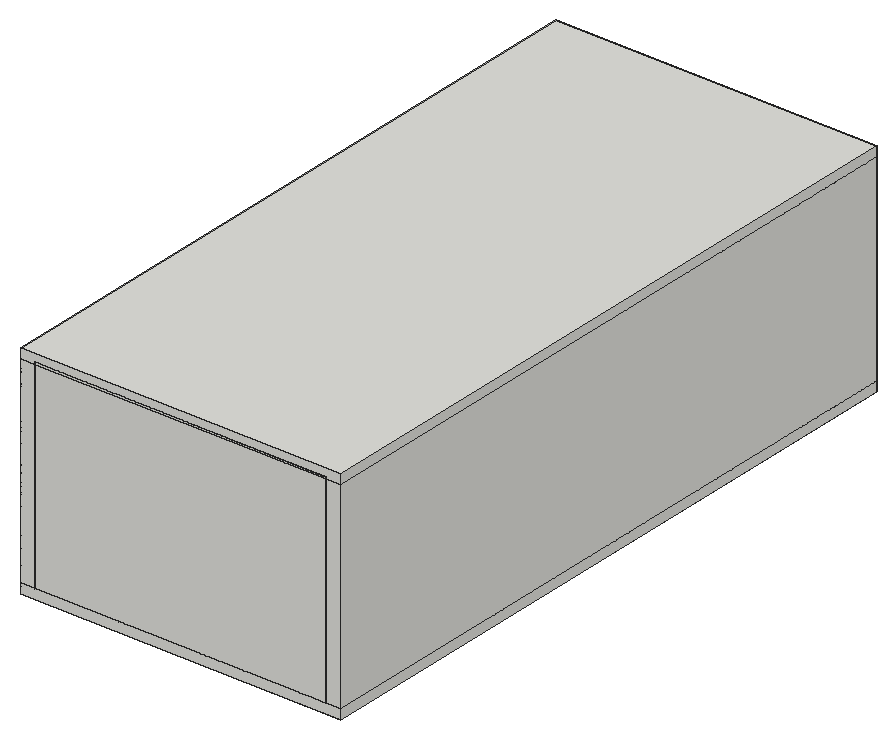
# SketchUp Ruby script. Lengths in inches.
U = 1.inch
M = Sketchup.active_model
def pt(a) = Geom::Point3d.new(a.map { |v| v * U })
def face(e, loops, mat)
  f = e.add_face(loops[0].map { |a| pt(a) })
  loops[1..].each { |l| e.add_face(l.map { |a| pt(a) }).erase! }
  f.material = f.back_material = mat if mat
  f
end
# faces: each face lists its corners as indices into pts; further lists are holes
def faces(e, pts, list, mat = nil) = list.each { |f| face(e, (f[0].is_a?(Array) ? f : [f]).map { |l| l.map { |i| pts[i] } }, mat) }
# xy, xz, yz: faces in a plane at the given z, y or x. An outline is a flat list of corners, or four numbers for a rectangle; further outlines are holes
def ring(l) = l.size == 4 ? [[l[0], l[1]], [l[2], l[1]], [l[2], l[3]], [l[0], l[3]]] : l.each_slice(2).to_a
def flat(e, list, mat, &to3) = list.each { |f| face(e, (f[0].is_a?(Array) ? f : [f]).map { |l| ring(l).map { |u, v| to3.(u, v) } }, mat) }
def xy(e, z, list, mat = nil) = flat(e, list, mat) { |x, y| [x, y, z] }
def xz(e, y, list, mat = nil) = flat(e, list, mat) { |x, z| [x, y, z] }
def yz(e, x, list, mat = nil) = flat(e, list, mat) { |y, z| [x, y, z] }
def lines(e, pts, list) = list.each { |a, b| e.add_line(pt(pts[a]), pt(pts[b])) }
# prism: a flat outline (further loops are holes) pulled along v
def prism(e, loops, v, mat = nil)
  f = face(e, loops, mat); d = Geom::Vector3d.new(v.map { |x| x * U })
  f.pushpull(f.normal.samedirection?(d) ? d.length : -d.length)
end
def box(e, o, s, mat = nil) = prism(e, [[o, [o[0] + s[0], o[1], o[2]], [o[0] + s[0], o[1] + s[1], o[2]], [o[0], o[1] + s[1], o[2]]]], [0, 0, s[2]], mat)
def at(x, y, z, deg = 0) = Geom::Transformation.translation(pt([x, y, z])) * Geom::Transformation.rotation(ORIGIN, Z_AXIS, deg.degrees)
def axes(o, x, y, z) = Geom::Transformation.new([*x, 0, *y, 0, *z, 0, *pt(o).to_a, 1])
def part(name) = M.definitions.add(name)
# library, detail: a bought-in or finely detailed component or shape, given as its bounding box
def library(name, o, s) = part(name).tap { |d| box(d.entities, o, s) }
def detail(e, o, s) = box(e.add_group.entities, o, s)
def put(e, d, t, mat = nil) = e.add_instance(d, t).tap { |i| i.material = mat if mat }
def group(e, t, mat = nil) = e.add_group.tap { |g| g.transformation = t; g.material = mat if mat }.entities
root = M.entities
M.materials.add("Emissive").color = [238, 234, 167]
M.materials.add("Generic").color = [144, 152, 143]
M.materials.add("Generic\#1").color = [229, 227, 227]
M.materials.add("Gold 10k").color = [251, 232, 180]
M.materials.add("Granite I 80cm").color = [116, 119, 117]
M.materials.add("Marble White 100cm").color = [222, 222, 222]
M.materials.add("[Color M07]").color = [58, 58, 58]
M.materials.add("[Wood Floor Light]").color = [204, 176, 127]
c1 = library("Appliance 143 028",[-10.4,-8.7,0],[20.81,17.4,15.71])
c2 = library("Kitchen Sink 180 028",[-24.73,-12.25,-4.96],[49.46,27.83,19.44])
c3 = library("Refrigerator 300 009",[-13.27,-13.92,-0.16],[26.54,24.77,79.78])
c4 = library("Pendant 16-22",[-19.69,-1.32,-27.17],[39.38,2.64,27.17])
c5 = library("Vase 014",[-3.77,-3.77,0],[7.54,7.54,8.49])
c6 = library("Peperomia 450 001",[-6.6875,-10.1875,-9.42],[16.7,12.74,19.03])
c7 = library("Vase 008",[-10.64,-10.96,0.22],[21.74,21.78,17.78])
c8 = library("Potted Plant 50-23",[-3.4,-3.5,0],[6.8,7,9.93])
c9 = library("Potted Plant 50-24",[-2.18,-2.1,0],[4.36,4.2,6.7])
c10 = library("Granadilla 71-16",[-5.43,-5.43,0],[10.86,10.86,6.68])
c11 = library("Chimney",[0,-14.34,0],[33.95,14.34,33.72])
c12 = library("Группа\#68",[0,0,-0.08],[23.6,20.47,1.99])
c13 = part("варочная панель")
p = [[285.71,355.65,85.04],[285.71,355.46,84.84]]
lines(c13.entities,p,[[0,1]])
put(c13.entities,c12,at(-9.77,-7.47,0.71))
c14 = library("kitchen utensils",[9.35,268.74,61.77],[151.43,198.45,25.1])
c15 = library("UTENCILIOS",[-3.38,-3.35,0],[5.31,6.7,10.38])
c16 = library("DCDH",[-31.47,375.85,61.79],[133.92,11.04,35.38])
c17 = library("JSilva Jalousie",[-31.89,-0.05,0.1],[63.78,4.97,70.86])
c18 = library("Handle_13.skp\#1",[-2.33,-0.79,-0.19],[4.66,0.79,0.38])
c19 = library("Tlon Light 1950 Ceiling 152 010",[-38.39,-38.39,-3.78],[76.78,76.78,3.41])
c20 = library("Tlon Cubo 860 Ceiling 152 005",[-16.93,-16.93,-3.79],[33.86,33.86,3.79])
xy(root,-6,[[0,0,198,413.6875]])
xy(root,0,[[0,0,9,0,9,404.6875,189,404.6875,189,0,198,0,198,413.6875,0,413.6875],[9,198.68,9,404.6875,33,404.6875,33,384.6875,29,384.6875,29,198.68],[169,235.17,189,380.6875],[169,380.6875,169,384.6875,33,384.6875,33,404.6875,189,404.6875,189,380.6875]])
xy(root,0,[[9,0,189,0,189,235.17,169,235.17,169,384.6875,29,384.6875,29,198.68,9,198.68]],"Marble White 100cm")
xy(root,4,[[29,217.0625,32.25,217.46],[29,239.13,32.25,239.53],[165.75,259.03,169,259.43],[165.75,283.28,169,283.68],[165.75,307.53,169,307.93],
  [29,325.52,32.25,325.92],[165.75,331.78,169,332.18],[165.75,356.04,169,356.44],[29,380.6875,33,384.6875],[33,380.6875,34.83,384.6875],
  [34.83,381.4375,35.23,384.6875],[73.14,381.4375,73.54,384.6875],[136.65,381.4375,137.05,384.6875],[160.91,381.4375,161.31,384.6875]])
xy(root,4,[[9,194.68,29,198.68],[29,194.68,33,217.0625],[29,217.46,33,239.13],[165,235.17,169,259.03],[29,239.53,33,325.52],
  [165,259.43,169,283.28],[165,283.68,169,307.53],[165,307.93,169,331.78],[29,325.92,33,380.6875],[165,332.18,169,356.04],
  [165,356.44,169,380.6875],[35.23,380.6875,54.1875,384.6875],[54.59,380.6875,73.14,384.6875],[73.54,380.6875,136.65,384.6875],[137.05,380.6875,160.91,384.6875],
  [161.31,380.6875,169,384.6875],[54.1875,381.4375,54.59,384.6875]],"[Color M07]")
xy(root,14.31,[[73.54,380.6875,136.65,381.4375]],"Gold 10k")
xy(root,14.57,[[32.25,239.53,33,325.52]],"Gold 10k")
xy(root,14.71,[[73.54,380.6875,136.65,381.4375]],"Gold 10k")
xy(root,14.97,[[32.25,239.53,33,325.52]],"Gold 10k")
xy(root,25.01,[[73.54,380.6875,136.65,381.4375]],"Gold 10k")
xy(root,25.41,[[73.54,380.6875,136.65,381.4375]],"Gold 10k")
xy(root,25.54,[[32.25,239.53,33,325.52]],"Gold 10k")
xy(root,25.94,[[32.25,239.53,33,325.52]],"Gold 10k")
xy(root,33,[[9,194.68,9,404.6875,33,404.6875,33,381.4375,32.25,381.4375,32.25,194.68],[165.75,235.17,189,380.6875],[165.75,380.6875,165.75,381.4375,33,381.4375,33,404.6875,189,404.6875,189,380.6875]])
xy(root,33,[[32.25,194.68,33,217.0625],[32.25,217.46,33,239.13],[165,235.17,165.75,259.03],[32.25,239.53,33,325.52],[165,259.43,165.75,283.28],
  [165,283.68,165.75,307.53],[165,307.93,165.75,331.78],[32.25,325.92,33,380.6875],[165,332.18,165.75,356.04],[165,356.44,165.75,380.6875],
  [32.25,380.6875,33,381.4375],[33,380.6875,34.83,381.4375],[35.23,380.6875,54.1875,381.4375],[54.59,380.6875,73.14,381.4375],[73.54,380.6875,136.65,381.4375],
  [137.05,380.6875,160.91,381.4375],[161.31,380.6875,165,381.4375],[165,380.6875,165.75,381.4375]],"[Color M07]")
xy(root,34,[[9,194.68,9,404.6875,33,404.6875,33,381.4375,32.25,381.4375,32.25,194.68],[165.75,235.17,189,380.6875],[165.75,380.6875,165.75,381.4375,33,381.4375,33,404.6875,189,404.6875,189,380.6875],[163,380.6875,165.75,381.4375]])
xy(root,34,[[9,192.68,35,194.68],[32.25,194.68,35,378.6875],[163,235.17,165.75,380.6875],[32.25,378.6875,33,381.4375],[33,378.6875,163,381.4375]],"Granite I 80cm")
xy(root,36,[[9,192.68,35,192.68,35,378.6875,33,378.6875,33,404.6875,9,404.6875],[163,235.17,189,380.6875],[33,378.6875,163,378.6875,163,380.6875,189,380.6875,189,404.6875,33,404.6875]],"Granite I 80cm")
xy(root,46.2,[[76.15,404.6875,143.46,413.6875]])
xy(root,60,[[9,194.68,11,208.52],[187,235,189,386.6875],[9,291.08,11,386.6875],[9,386.6875,11,404.6875],[187,386.6875,189,404.6875],
  [11,402.6875,69.27,404.6875],[151.97,402.6875,187,404.6875]],"Emissive")
xy(root,60,[[11,194.68,27,208.52],[171,235,171,272.52,171.75,272.52,171.75,272.92,171,272.92,171,310.44,171.75,310.44,171.75,310.84,171,310.84,171,348.37,171.75,348.37,171.75,348.77,171,348.77,171,386.6875,187,386.6875,187,235],[11,291.08,11,386.6875,27,386.6875,27,339.09,26.25,339.09,26.25,338.69,27,338.69,27,291.08],[11,386.6875,69.27,402.6875],[151.97,386.6875,187,402.6875]],"[Wood Floor Light]")
xy(root,61.79,[[28.79,386.6875,46.04,402.6875],[49.61,386.6875,67.49,402.6875]],"[Wood Floor Light]")
xy(root,61.83,[[10.83,194.68,25.17,206.99]],"[Wood Floor Light]")
xy(root,62.1,[[154.07,386.6875,168.9,402.6875]],"[Wood Floor Light]")
xy(root,70.51,[[28.79,400.6875,46.04,402.6875],[49.61,400.6875,67.49,402.6875]],"Emissive")
xy(root,70.51,[[28.79,386.6875,46.04,400.6875],[49.61,386.6875,67.49,400.6875]],"[Wood Floor Light]")
xy(root,71.74,[[28.79,386.6875,46.04,402.6875],[49.61,386.6875,67.49,402.6875]],"[Wood Floor Light]")
xy(root,75.07,[[10.83,204.99,25.17,206.99]],"Emissive")
xy(root,75.07,[[10.83,194.68,25.17,204.99]],"[Wood Floor Light]")
xy(root,75.16,[[154.07,400.6875,168.9,402.6875]],"Emissive")
xy(root,75.16,[[154.07,386.6875,168.9,400.6875]],"[Wood Floor Light]")
xy(root,76.45,[[10.83,194.68,25.17,206.99],[154.07,386.6875,168.9,402.6875]],"[Wood Floor Light]")
xy(root,78.88,[[28.79,400.6875,46.04,402.6875]],"Emissive")
xy(root,78.88,[[28.79,386.6875,46.04,400.6875]],"[Wood Floor Light]")
xy(root,79.26,[[49.61,400.6875,67.49,402.6875]],"Emissive")
xy(root,79.26,[[49.61,386.6875,67.49,400.6875]],"[Wood Floor Light]")
xy(root,80.12,[[28.79,386.6875,46.04,402.6875]],"[Wood Floor Light]")
xy(root,80.49,[[49.61,386.6875,67.49,402.6875]],"[Wood Floor Light]")
xy(root,85.27,[[76.15,404.6875,143.46,413.6875]])
xy(root,87.72,[[49.61,399.6875,67.49,402.6875],[28.79,400.6875,46.04,402.6875]],"Emissive")
xy(root,87.72,[[28.79,386.6875,46.04,400.6875],[49.61,386.6875,67.49,399.6875]],"[Wood Floor Light]")
xy(root,89.01,[[10.83,204.99,25.17,206.99]],"Emissive")
xy(root,89.01,[[10.83,194.68,25.17,204.99]],"[Wood Floor Light]")
xy(root,89.5,[[171,235,189,235,189,386.6875,171,386.6875,171,354.6875,171.75,354.6875,171.75,354.29,171,354.29,171,348.77,171.75,348.77,171.75,348.37,171,348.37,171,322.6875,171.75,322.6875,171.75,322.29,171,322.29,171,310.84,171.75,310.84,171.75,310.44,171,310.44,171,290.6875,171.75,290.6875,171.75,290.29,171,290.29,171,272.92,171.75,272.92,171.75,272.52,171,272.52,171,258.6875,171.75,258.6875,171.75,258.29,171,258.29],[171,258.29,171.75,258.6875],[9,386.6875,47.83,386.6875,47.83,387.4375,48.23,387.4375,48.23,386.6875,68.66,386.6875,68.66,387.4375,69.06,387.4375,69.06,386.6875,69.27,386.6875,69.27,404.6875,9,404.6875],[47.83,386.6875,48.23,387.4375],[68.66,386.6875,69.06,387.4375]])
xy(root,89.5,[[69.27,386.6875,69.27,404.6875,151.97,404.6875,151.97,386.6875,131.54,386.6875,131.54,387.4375,131.14,387.4375,131.14,386.6875,110.71,386.6875,110.71,387.4375,110.3125,387.4375,110.3125,386.6875,89.89,386.6875,89.89,387.4375,89.49,387.4375,89.49,386.6875]],"Generic")
xy(root,89.5,[[171,272.52,171.75,272.92],[171,290.29,171.75,290.6875],[171,310.44,171.75,310.84],[171,322.29,171.75,322.6875],[171,348.37,171.75,348.77],
  [171,354.29,171.75,354.6875]],"Gold 10k")
xy(root,89.5,[[171,194.6875,171,226.29,171.75,226.29,171.75,226.6875,171,226.6875,171,235,189,235,189,194.6875]],"[Wood Floor Light]")
xy(root,90.34,[[154.07,400.6875,168.9,402.6875]],"Emissive")
xy(root,90.34,[[154.07,386.6875,168.9,400.6875]],"[Wood Floor Light]")
xy(root,90.39,[[10.83,194.68,25.17,206.99]],"[Wood Floor Light]")
xy(root,91.64,[[154.07,386.6875,168.9,402.6875]],"[Wood Floor Light]")
xy(root,96,[[9,291.08,27,291.08,27,338.69,26.25,338.69,26.25,339.09,27,339.09,27,386.6875,9,386.6875],[9,386.6875,27,404.6875]])
xy(root,96,[[9,208.52,9,291.08,26.25,291.08,26.25,290.68,27,290.68,27,243.08,26.25,243.08,26.25,242.68,27,242.68,27,208.52]],"Generic")
xy(root,102.41,[[154.07,400.6875,168.9,402.6875]],"Emissive")
xy(root,102.41,[[154.07,386.6875,168.9,400.6875]],"[Wood Floor Light]")
xy(root,102.82,[[10.83,204.99,25.17,206.99]],"Emissive")
xy(root,102.82,[[10.83,194.68,25.17,204.99]],"[Wood Floor Light]")
xy(root,103.7,[[154.07,386.6875,168.9,402.6875]],"[Wood Floor Light]")
xy(root,104.2,[[10.83,194.68,25.17,206.99]],"[Wood Floor Light]")
xy(root,117.9,[[154.07,401.8125,168.9,402.6875]],"Emissive")
xy(root,117.9,[[154.07,386.6875,168.9,401.8125]],"[Wood Floor Light]")
xy(root,118.17,[[10.83,204.99,25.17,206.99]],"Emissive")
xy(root,118.17,[[10.83,194.68,25.17,204.99]],"[Wood Floor Light]")
xy(root,120,[[171.75,194.6875,189,386.6875],[9,195.43,9,404.6875,27,404.6875,27,387.4375,26.25,387.4375,26.25,195.43],[171.75,386.6875,171.75,387.4375,27,387.4375,27,404.6875,189,404.6875,189,386.6875]])
xy(root,120,[[9,194.68,26.25,195.43],[26.25,194.68,27,242.68],[171,194.6875,171.75,226.29],[171,226.6875,171.75,258.29],[26.25,243.08,27,290.68],
  [171,258.6875,171.75,290.29],[171,290.6875,171.75,322.29],[26.25,291.08,27,338.69],[171,322.6875,171.75,354.29],[26.25,339.09,27,387.4375],
  [171,354.6875,171.75,386.6875],[27,386.6875,47.83,387.4375],[48.23,386.6875,68.66,387.4375],[69.06,386.6875,89.49,387.4375],[89.89,386.6875,110.3125,387.4375],
  [110.71,386.6875,131.14,387.4375],[131.54,386.6875,151.97,387.4375],[151.97,386.6875,171.75,387.4375]],"[Color M07]")
xy(root,120.6875,[[171.75,194.6875,189,386.6875],[9,195.43,9,404.6875,27,404.6875,27,387.4375,26.25,387.4375,26.25,195.43],[171.75,386.6875,171.75,387.4375,27,387.4375,27,404.6875,189,404.6875,189,386.6875]])
xy(root,120.6875,[[9,194.68,26.25,195.43],[26.25,194.68,27,387.4375],[171,194.6875,171.75,386.6875],[27,386.6875,171.75,387.4375]],"[Color M07]")
xy(root,124,[[0,0,0,413.6875,198,413.6875,198,0,189,0,189,404.6875,9,404.6875,9,0],[9,0,189,155.6875],[9,194.68,27,404.6875],[171,194.6875,189,386.6875],[27,386.6875,189,404.6875]])
xy(root,124,[[[9,155.6875,9,194.68,27,194.68,27,386.6875,171,386.6875,171,194.6875,189,194.6875,189,155.6875],[52.375,181.0625,145.625,361.3125]]],"Generic\#1")
xy(root,124,[[79.36,208.04,118.64,334.33]],"[Wood Floor Light]")
xy(root,125.4375,[[9,0,189,155.6875],[[9,155.6875,189,155.6875,189,194.6875,171,194.6875,171,386.6875,27,386.6875,27,194.68,9,194.68],[51,179.6875,147,362.6875]],[80.73,208.04,117.27,332.96]])
xy(root,125.4375,[[51,179.6875,147,181.0625],[51,181.0625,52.375,362.6875],[145.625,181.0625,147,362.6875],[79.36,208.04,80.73,334.33],[117.27,208.04,118.64,334.33],
  [80.73,332.96,117.27,334.33],[52.375,361.3125,145.625,362.6875]],"Emissive")
xy(root,127.1875,[[[51,179.6875,147,362.6875],[80.73,208.04,117.27,332.96]]],"Generic\#1")
xy(root,130,[[0,0,198,413.6875]])
xz(root,0,[[0,-6,198,0],[0,0,9,124],[9,0,189,124],[189,0,198,124],[0,124,9,124,9,125.4375,189,125.4375,189,124,198,124,198,130,0,130],
  [9,124,189,125.4375]])
xz(root,155.6875,[[9,124,189,125.4375]])
xz(root,179.6875,[[51,125.4375,147,127.1875]],"Emissive")
xz(root,181.0625,[[52.375,124,145.625,125.4375]])
xz(root,192.68,[[9,34,35,36]],"Granite I 80cm")
xz(root,194.68,[[9,124,27,125.4375]])
xz(root,194.68,[[9,4,33,33]],"Generic")
xz(root,194.68,[[9,33,32.25,34],[[9,60,27,120],[10.83,61.83,25.17,118.17]],[9,120.6875,27,124]],"[Color M07]")
xz(root,194.68,[[10.83,75.07,25.17,76.45],[10.83,89.01,25.17,90.39],[10.83,102.82,25.17,104.2]],"[Wood Floor Light]")
xz(root,194.6875,[[171,124,189,125.4375]])
xz(root,194.6875,[[171,89.5,189,120]],"Generic")
xz(root,194.6875,[[171.75,120,189,120.6875],[171,120.6875,189,124]],"[Color M07]")
xz(root,195.43,[[9,120,26.25,120.6875]],"[Color M07]")
xz(root,198.68,[[9,0,29,4]],"[Color M07]")
xz(root,206.99,[[10.83,75.07,25.17,76.45],[10.83,89.01,25.17,90.39],[10.83,102.82,25.17,104.2]])
xz(root,206.99,[[10.83,61.83,25.17,75.07],[10.83,76.45,25.17,89.01],[10.83,90.39,25.17,102.82],[10.83,104.2,25.17,118.17]],"[Wood Floor Light]")
xz(root,208.04,[[80.73,125.4375,117.27,127.1875]],"Emissive")
xz(root,208.04,[[79.36,124,118.64,125.4375]],"[Wood Floor Light]")
xz(root,208.52,[[9,60,27,96]])
xz(root,217.0625,[[32.25,4,33,33]],"Gold 10k")
xz(root,217.46,[[32.25,4,33,33]],"Gold 10k")
xz(root,226.29,[[171,89.5,171.75,120]],"Gold 10k")
xz(root,226.6875,[[171,89.5,171.75,120]],"Gold 10k")
xz(root,235,[[171,60,189,89.5]])
xz(root,235.17,[[169,0,189,0,189,33,165,33,165,4,169,4]],"Generic")
xz(root,235.17,[[163,34,189,36]],"Granite I 80cm")
xz(root,235.17,[[165.75,33,189,34]],"[Color M07]")
xz(root,239.13,[[32.25,4,33,14.97],[32.25,14.97,33,25.94],[32.25,25.94,33,33]],"Gold 10k")
xz(root,239.53,[[32.25,4,33,14.57],[32.25,14.97,33,25.54],[32.25,25.94,33,33]],"Gold 10k")
xz(root,242.68,[[26.25,96,27,120]],"Gold 10k")
xz(root,243.08,[[26.25,96,27,120]],"Gold 10k")
xz(root,258.29,[[171,89.5,171.75,120]],"Gold 10k")
xz(root,258.6875,[[171,89.5,171.75,120]],"Gold 10k")
xz(root,259.03,[[165,4,165.75,33]],"Gold 10k")
xz(root,259.43,[[165,4,165.75,33]],"Gold 10k")
xz(root,272.52,[[171,60,171.75,89.5]],"Gold 10k")
xz(root,272.92,[[171,60,171.75,89.5]],"Gold 10k")
xz(root,283.28,[[165,4,165.75,33]],"Gold 10k")
xz(root,283.68,[[165,4,165.75,33]],"Gold 10k")
xz(root,290.29,[[171,89.5,171.75,120]],"Gold 10k")
xz(root,290.68,[[26.25,96,27,120]],"Gold 10k")
xz(root,290.6875,[[171,89.5,171.75,120]],"Gold 10k")
xz(root,291.08,[[26.25,96,27,120]],"Gold 10k")
xz(root,291.08,[[9,60,27,96]],"[Wood Floor Light]")
xz(root,307.53,[[165,4,165.75,33]],"Gold 10k")
xz(root,307.93,[[165,4,165.75,33]],"Gold 10k")
xz(root,310.44,[[171,60,171.75,89.5]],"Gold 10k")
xz(root,310.84,[[171,60,171.75,89.5]],"Gold 10k")
xz(root,322.29,[[171,89.5,171.75,120]],"Gold 10k")
xz(root,322.6875,[[171,89.5,171.75,120]],"Gold 10k")
xz(root,325.52,[[32.25,4,33,14.57],[32.25,14.97,33,25.54],[32.25,25.94,33,33]],"Gold 10k")
xz(root,325.92,[[32.25,4,33,14.97],[32.25,14.97,33,25.94],[32.25,25.94,33,33]],"Gold 10k")
xz(root,331.78,[[165,4,165.75,33]],"Gold 10k")
xz(root,332.18,[[165,4,165.75,33]],"Gold 10k")
xz(root,332.96,[[80.73,125.4375,117.27,127.1875]],"Emissive")
xz(root,334.33,[[79.36,124,118.64,125.4375]])
xz(root,338.69,[[26.25,60,27,96],[26.25,96,27,120]],"Gold 10k")
xz(root,339.09,[[26.25,60,27,96],[26.25,96,27,120]],"Gold 10k")
xz(root,348.37,[[171,60,171.75,89.5]],"Gold 10k")
xz(root,348.77,[[171,60,171.75,89.5]],"Gold 10k")
xz(root,354.29,[[171,89.5,171.75,120]],"Gold 10k")
xz(root,354.6875,[[171,89.5,171.75,120]],"Gold 10k")
xz(root,356.04,[[165,4,165.75,33]],"Gold 10k")
xz(root,356.44,[[165,4,165.75,33]],"Gold 10k")
xz(root,361.3125,[[52.375,124,145.625,125.4375]],"Generic\#1")
xz(root,362.6875,[[51,125.4375,147,127.1875]],"Emissive")
xz(root,378.6875,[[33,34,35,36]])
xz(root,378.6875,[[35,34,163,36]],"Granite I 80cm")
xz(root,380.6875,[[169,0,189,0,189,33,165,33,165,4,169,4],[165.75,33,189,34],[163,34,189,36]])
xz(root,380.6875,[[33,4,34.83,33],[35.23,4,54.1875,33],[54.59,4,73.14,33],[73.54,4,136.65,14.31],[137.05,4,160.91,33],
  [161.31,4,165,33],[73.54,14.71,136.65,25.01],[73.54,25.41,136.65,33]],"Generic")
xz(root,381.4375,[[34.83,4,35.23,33],[54.1875,4,54.59,33],[73.14,4,73.54,33],[136.65,4,137.05,33],[160.91,4,161.31,33],
  [73.54,14.31,136.65,14.71],[73.54,25.01,136.65,25.41]],"Gold 10k")
xz(root,381.4375,[[32.25,33,33,34],[33,33,165.75,34]],"[Color M07]")
xz(root,384.6875,[[29,0,33,4],[33,0,169,4]],"[Color M07]")
xz(root,386.6875,[[9,60,27,89.5],[171,60,189,89.5],[9,89.5,27,96],[171,89.5,189,120],[171.75,120,189,120.6875],
  [171,120.6875,189,124],[27,124,171,125.4375]])
xz(root,386.6875,[[27,89.5,47.83,120],[48.23,89.5,68.66,120],[69.06,89.5,89.49,120],[89.89,89.5,110.3125,120],[110.71,89.5,131.14,120],
  [131.54,89.5,151.97,120]],"Generic")
xz(root,386.6875,[[[27,60,47.83,89.5],[28.79,61.79,46.04,87.72]],[[47.83,60,69.27,89.5],[49.61,61.79,67.49,87.72]],[[151.97,60,171,120],[154.07,62.1,168.9,117.9]],[27,120.6875,171,124]],"[Color M07]")
xz(root,386.6875,[[28.79,70.51,46.04,71.74],[49.61,70.51,67.49,71.74],[154.07,75.16,168.9,76.45],[28.79,78.88,46.04,80.12],[49.61,79.26,67.49,80.49],
  [154.07,90.34,168.9,91.64],[154.07,102.41,168.9,103.7]],"[Wood Floor Light]")
xz(root,387.4375,[[47.83,89.5,48.23,120],[68.66,89.5,69.06,120],[89.49,89.5,89.89,120],[110.3125,89.5,110.71,120],[131.14,89.5,131.54,120]],"Gold 10k")
xz(root,387.4375,[[26.25,120,27,120.6875],[27,120,171.75,120.6875]],"[Color M07]")
xz(root,402.6875,[[28.79,70.51,46.04,71.74],[49.61,70.51,67.49,71.74],[154.07,75.16,168.9,76.45],[28.79,78.88,46.04,80.12],[49.61,79.26,67.49,80.49],
  [154.07,90.34,168.9,91.64],[154.07,102.41,168.9,103.7]])
xz(root,402.6875,[[28.79,61.79,46.04,70.51],[49.61,61.79,67.49,70.51],[154.07,62.1,168.9,75.16],[28.79,71.74,46.04,78.88],[49.61,71.74,67.49,79.26],
  [154.07,76.45,168.9,90.34],[28.79,80.12,46.04,87.72],[49.61,80.49,67.49,87.72],[154.07,91.64,168.9,102.41],[154.07,103.7,168.9,117.9]],"[Wood Floor Light]")
xz(root,404.6875,[[9,0,33,33],[33,0,189,33],[9,33,33,34],[33,33,189,34],[9,34,33,36],
  [33,34,189,36],[151.97,60,151.97,89.5,9,89.5,9,96,27,96,27,120,189,120,189,60],[9,60,69.27,89.5],[9,96,27,120],[9,120,27,120.6875],
  [27,120,189,120.6875],[9,120.6875,27,124],[27,120.6875,189,124]])
xz(root,404.6875,[[[9,36,189,36,189,60,151.97,60,151.97,89.5,69.27,89.5,69.27,60,9,60],[76.15,46.2,143.46,85.27]]],"Granite I 80cm")
xz(root,413.6875,[[0,-6,198,0],[[0,0,198,124],[76.15,46.2,143.46,85.27]],[0,124,198,130]])
yz(root,0,[[0,-6,413.6875,0],[0,0,413.6875,124],[0,124,413.6875,130]])
yz(root,9,[[198.68,0,404.6875,0,404.6875,33,194.68,33,194.68,4,198.68,4],[194.68,33,404.6875,34],[192.68,34,404.6875,36],[194.68,60,208.52,96],[291.08,60,386.6875,96],
  [386.6875,60,404.6875,89.5],[386.6875,89.5,404.6875,96],[194.68,96,404.6875,120],[195.43,120,404.6875,120.6875],[194.68,120.6875,404.6875,124],
  [0,124,155.6875,125.4375],[155.6875,124,194.68,125.4375]])
yz(root,9,[[0,0,198.68,0,198.68,4,194.68,4,194.68,34,192.68,34,192.68,36,404.6875,36,404.6875,60,291.08,60,291.08,96,208.52,96,208.52,60,194.68,60,194.68,120,195.43,120,195.43,120.6875,194.68,120.6875,194.68,124,0,124]],"Granite I 80cm")
yz(root,10.83,[[194.68,75.07,206.99,76.45],[194.68,89.01,206.99,90.39],[194.68,102.82,206.99,104.2]])
yz(root,10.83,[[194.68,61.83,206.99,75.07],[194.68,76.45,206.99,89.01],[194.68,90.39,206.99,96],[194.68,96,206.99,102.82],[194.68,104.2,206.99,118.17]],"[Wood Floor Light]")
yz(root,25.17,[[194.68,75.07,206.99,76.45],[194.68,89.01,206.99,90.39],[194.68,102.82,206.99,104.2]])
yz(root,25.17,[[194.68,61.83,206.99,75.07],[194.68,76.45,206.99,89.01],[194.68,90.39,206.99,96],[194.68,96,206.99,102.82],[194.68,104.2,206.99,118.17]],"[Wood Floor Light]")
yz(root,26.25,[[338.69,60,339.09,96],[242.68,96,243.08,120],[290.68,96,291.08,120],[338.69,96,339.09,120]],"Gold 10k")
yz(root,26.25,[[195.43,120,387.4375,120.6875]],"[Color M07]")
yz(root,27,[[386.6875,96,404.6875,120],[387.4375,120,404.6875,120.6875],[386.6875,120.6875,404.6875,124],[194.68,124,386.6875,125.4375]])
yz(root,27,[[194.68,60,208.52,96],[291.08,60,338.69,96],[339.09,60,386.6875,96],[194.68,96,242.68,120],[243.08,96,290.68,120],
  [291.08,96,338.69,120],[339.09,96,386.6875,120]],"Generic")
yz(root,27,[[194.68,120.6875,386.6875,124]],"[Color M07]")
yz(root,28.79,[[386.6875,70.51,402.6875,71.74],[386.6875,78.88,402.6875,80.12]])
yz(root,28.79,[[386.6875,61.79,402.6875,70.51],[386.6875,71.74,402.6875,78.88],[386.6875,80.12,402.6875,87.72]],"[Wood Floor Light]")
yz(root,29,[[380.6875,0,384.6875,4]])
yz(root,29,[[198.68,0,380.6875,4]],"[Color M07]")
yz(root,32.25,[[217.0625,4,217.46,33],[239.13,4,239.53,33],[325.52,4,325.92,33],[239.53,14.57,325.52,14.97],[239.53,25.54,325.52,25.94]],"Gold 10k")
yz(root,32.25,[[194.68,33,381.4375,34]],"[Color M07]")
yz(root,33,[[384.6875,0,404.6875,0,404.6875,33,380.6875,33,380.6875,4,384.6875,4],[381.4375,33,404.6875,34],[378.6875,34,404.6875,36]])
yz(root,33,[[194.68,4,217.0625,33],[217.46,4,239.13,33],[239.53,4,325.52,14.57],[325.92,4,380.6875,33],[239.53,14.97,325.52,25.54],
  [239.53,25.94,325.52,33]],"Generic")
yz(root,34.83,[[380.6875,4,381.4375,33]],"Gold 10k")
yz(root,35,[[192.68,34,378.6875,36]],"Granite I 80cm")
yz(root,35.23,[[380.6875,4,381.4375,33]],"Gold 10k")
yz(root,46.04,[[386.6875,70.51,402.6875,71.74],[386.6875,78.88,402.6875,80.12]])
yz(root,46.04,[[386.6875,61.79,402.6875,70.51],[386.6875,71.74,402.6875,78.88],[386.6875,80.12,402.6875,87.72]],"[Wood Floor Light]")
yz(root,47.83,[[386.6875,89.5,387.4375,120]],"Gold 10k")
yz(root,48.23,[[386.6875,89.5,387.4375,120]],"Gold 10k")
yz(root,49.61,[[386.6875,70.51,402.6875,71.74],[386.6875,79.26,402.6875,80.49]])
yz(root,49.61,[[386.6875,61.79,402.6875,70.51],[386.6875,71.74,402.6875,79.26],[386.6875,80.49,402.6875,87.72]],"[Wood Floor Light]")
yz(root,51,[[179.6875,125.4375,362.6875,127.1875]],"Emissive")
yz(root,52.375,[[181.0625,124,361.3125,125.4375]],"Generic\#1")
yz(root,54.1875,[[380.6875,4,381.4375,33]],"Gold 10k")
yz(root,54.59,[[380.6875,4,381.4375,33]],"Gold 10k")
yz(root,67.49,[[386.6875,70.51,402.6875,71.74],[386.6875,79.26,402.6875,80.49]])
yz(root,67.49,[[386.6875,61.79,402.6875,70.51],[386.6875,71.74,402.6875,79.26],[386.6875,80.49,402.6875,87.72]],"[Wood Floor Light]")
yz(root,68.66,[[386.6875,89.5,387.4375,120]],"Gold 10k")
yz(root,69.06,[[386.6875,89.5,387.4375,120]],"Gold 10k")
yz(root,69.27,[[386.6875,60,404.6875,89.5]],"Generic")
yz(root,73.14,[[380.6875,4,381.4375,14.71],[380.6875,14.71,381.4375,25.41],[380.6875,25.41,381.4375,33]],"Gold 10k")
yz(root,73.54,[[380.6875,25.41,381.4375,33]])
yz(root,73.54,[[380.6875,4,381.4375,14.31],[380.6875,14.71,381.4375,25.01]],"Gold 10k")
yz(root,76.15,[[404.6875,46.2,413.6875,85.27]])
yz(root,79.36,[[208.04,124,334.33,125.4375]],"[Wood Floor Light]")
yz(root,80.73,[[208.04,125.4375,332.96,127.1875]],"Emissive")
yz(root,89.49,[[386.6875,89.5,387.4375,120]],"Gold 10k")
yz(root,89.89,[[386.6875,89.5,387.4375,120]],"Gold 10k")
yz(root,110.3125,[[386.6875,89.5,387.4375,120]],"Gold 10k")
yz(root,110.71,[[386.6875,89.5,387.4375,120]],"Gold 10k")
yz(root,117.27,[[208.04,125.4375,332.96,127.1875]],"Emissive")
yz(root,118.64,[[208.04,124,334.33,125.4375]],"[Wood Floor Light]")
yz(root,131.14,[[386.6875,89.5,387.4375,120]],"Gold 10k")
yz(root,131.54,[[386.6875,89.5,387.4375,120]],"Gold 10k")
yz(root,136.65,[[380.6875,4,381.4375,14.31],[380.6875,14.71,381.4375,25.01],[380.6875,25.41,381.4375,33]],"Gold 10k")
yz(root,137.05,[[380.6875,4,381.4375,14.71],[380.6875,14.71,381.4375,25.41],[380.6875,25.41,381.4375,33]],"Gold 10k")
yz(root,143.46,[[404.6875,46.2,413.6875,85.27]])
yz(root,145.625,[[181.0625,124,361.3125,125.4375]],"Generic\#1")
yz(root,147,[[179.6875,125.4375,362.6875,127.1875]],"Emissive")
yz(root,151.97,[[386.6875,60,404.6875,89.5]],"Generic")
yz(root,154.07,[[386.6875,75.16,402.6875,76.45],[386.6875,90.34,402.6875,91.64],[386.6875,102.41,402.6875,103.7]])
yz(root,154.07,[[386.6875,62.1,402.6875,75.16],[386.6875,76.45,402.6875,89.5],[386.6875,89.5,402.6875,90.34],[386.6875,91.64,402.6875,102.41],[386.6875,103.7,402.6875,117.9]],"[Wood Floor Light]")
yz(root,160.91,[[380.6875,4,381.4375,33]],"Gold 10k")
yz(root,161.31,[[380.6875,4,381.4375,33]],"Gold 10k")
yz(root,163,[[378.6875,34,380.6875,36]])
yz(root,163,[[235.17,34,378.6875,36]],"Granite I 80cm")
yz(root,165,[[235.17,4,259.03,33],[259.43,4,283.28,33],[283.68,4,307.53,33],[307.93,4,331.78,33],[332.18,4,356.04,33],
  [356.44,4,380.6875,33]],"Generic")
yz(root,165.75,[[259.03,4,259.43,33],[283.28,4,283.68,33],[307.53,4,307.93,33],[331.78,4,332.18,33],[356.04,4,356.44,33]],"Gold 10k")
yz(root,165.75,[[235.17,33,380.6875,34],[380.6875,33,381.4375,34]],"[Color M07]")
yz(root,168.9,[[386.6875,75.16,402.6875,76.45],[386.6875,90.34,402.6875,91.64],[386.6875,102.41,402.6875,103.7]])
yz(root,168.9,[[386.6875,62.1,402.6875,75.16],[386.6875,76.45,402.6875,89.5],[386.6875,89.5,402.6875,90.34],[386.6875,91.64,402.6875,102.41],[386.6875,103.7,402.6875,117.9]],"[Wood Floor Light]")
yz(root,169,[[235.17,0,380.6875,4],[380.6875,0,384.6875,4]],"[Color M07]")
yz(root,171,[[194.6875,124,386.6875,125.4375]])
yz(root,171,[[235,60,272.52,89.5],[272.92,60,310.44,89.5],[310.84,60,348.37,89.5],[348.77,60,386.6875,89.5],[194.6875,89.5,226.29,120],
  [226.6875,89.5,258.29,120],[258.6875,89.5,290.29,120],[290.6875,89.5,322.29,120],[322.6875,89.5,354.29,120],[354.6875,89.5,386.6875,120]],"Generic")
yz(root,171,[[194.6875,120.6875,386.6875,124]],"[Color M07]")
yz(root,171.75,[[272.52,60,272.92,89.5],[310.44,60,310.84,89.5],[348.37,60,348.77,89.5],[226.29,89.5,226.6875,120],[258.29,89.5,258.6875,120],
  [290.29,89.5,290.6875,120],[322.29,89.5,322.6875,120],[354.29,89.5,354.6875,120]],"Gold 10k")
yz(root,171.75,[[194.6875,120,386.6875,120.6875],[386.6875,120,387.4375,120.6875]],"[Color M07]")
yz(root,189,[[235.17,0,380.6875,33],[380.6875,0,404.6875,33],[235.17,33,380.6875,34],[380.6875,33,404.6875,34],[235.17,34,380.6875,36],
  [380.6875,34,404.6875,36],[235,60,386.6875,89.5],[386.6875,60,404.6875,120],[194.6875,89.5,386.6875,120],[194.6875,120,386.6875,120.6875],
  [386.6875,120,404.6875,120.6875],[194.6875,120.6875,386.6875,124],[386.6875,120.6875,404.6875,124],[0,124,155.6875,125.4375],[155.6875,124,194.6875,125.4375]])
yz(root,189,[[0,0,0,124,194.6875,124,194.6875,89.5,235,89.5,235,60,404.6875,60,404.6875,36,235.17,36,235.17,0]],"Granite I 80cm")
yz(root,198,[[0,-6,413.6875,0],[0,0,413.6875,124],[0,124,413.6875,130]])
p = [[33,325.52,25.55],[33,325.62,25.55],[33,325.52,14.58],[33,325.62,14.58]]
lines(root,p,[[0,1],[2,3]])
put(root,c1,at(19.54,294.64,36))
put(root,c2,axes([105.35,391.33,36],[0.89,0,0],[0,0.6954,0],[0,0,1]))
put(root,c3,axes([177.17,214.24,0.02],[0,-1,0],[1,0,0],[0,0,1.12]))
put(root,c4,at(98.43,276.77,124))
put(root,c5,at(21.41,198.44,76.45))
put(root,c6,at(17.45,200.16,104.2))
put(root,c7,at(174.92,386.1,36))
put(root,c8,at(19.59,393.97,36))
put(root,c8,at(14.4,199.97,76.45))
put(root,c8,at(11.84,212.79,36))
put(root,c8,at(163.56,394.23,36))
put(root,c9,at(25.9,398.46,36))
put(root,c10,at(47.9375,388.81,36))
put(root,c11,axes([12.66,219.07,62.28],[0,2.12128,0],[-1,0,0],[0,0,1]))
put(root,c13,axes([23.38,251.18,35.37],[0,2.25,0],[-1,0,0],[0,0,1]))
put(root,c14,at(4.75,-72.5,0))
put(root,c15,at(17.54,217.5,36))
put(root,c16,at(65.28,13.27,0))
put(root,c6,at(161.18,392.17,103.79))
put(root,c5,at(21.41,198.44,90.39))
put(root,c5,at(14.23,198.44,90.39))
put(root,c17,axes([109.8,409.24,46.15],[1.05539,0,0],[0,1,0],[0,0,0.55122]))
put(root,c18,axes([102.59,380.6875,29.78],[3.06,0,0],[0,2.48,0],[0,0,2]))
put(root,c18,axes([102.59,380.6875,20.65],[3.06,0,0],[0,2.48,0],[0,0,2]))
put(root,c18,axes([102.59,380.6875,11.28],[3.06,0,0],[0,2.48,0],[0,0,2]))
put(root,c18,axes([33,268.16,29.0625],[0,3.06,0],[-2.48,0,0],[0,0,2]))
put(root,c18,axes([139.14,380.6875,27.09],[0,0,1.7748],[0,2.48,0],[-2,0,0]))
put(root,c18,axes([69.14,380.6875,27.09],[0,0,1.7748],[0,2.48,0],[-2,0,0]))
put(root,c18,axes([49.77,380.6875,27.09],[0,0,1.7748],[0,2.48,0],[-2,0,0]))
put(root,c18,axes([44.87,386.6875,97.31],[0,0,1.7748],[0,2.48,0],[-2,0,0]))
put(root,c18,axes([51.12,386.6875,97.31],[0,0,1.7748],[0,2.48,0],[-2,0,0]))
put(root,c18,axes([92.87,386.6875,97.31],[0,0,1.7748],[0,2.48,0],[-2,0,0]))
put(root,c18,axes([86.62,386.6875,97.31],[0,0,1.7748],[0,2.48,0],[-2,0,0]))
put(root,c18,axes([134.68,386.6875,97.31],[0,0,1.7748],[0,2.48,0],[-2,0,0]))
put(root,c18,axes([128.43,386.6875,97.31],[0,0,1.7748],[0,2.48,0],[-2,0,0]))
put(root,c18,axes([33,268.16,20.6875],[0,3.06,0],[-2.48,0,0],[0,0,2]))
put(root,c18,axes([33,268.16,11.375],[0,3.06,0],[-2.48,0,0],[0,0,2]))
put(root,c18,axes([33,211.84,25.38],[0,0,1.7748],[-2.48,0,0],[0,-2,0]))
put(root,c18,axes([33,221.34,25.38],[0,0,1.7748],[-2.48,0,0],[0,-2,0]))
put(root,c18,axes([33,332.22,25.38],[0,0,1.7748],[-2.48,0,0],[0,-2,0]))
put(root,c18,axes([27,345.78,106.1],[0,0,1.7748],[-2.48,0,0],[0,-2,0]))
put(root,c18,axes([27,237.21,106.1],[0,0,1.7748],[-2.48,0,0],[0,-2,0]))
put(root,c18,axes([27,246.9,106.1],[0,0,1.7748],[-2.48,0,0],[0,-2,0]))
put(root,c18,axes([27,326.4,106.1],[0,0,1.7748],[-2.48,0,0],[0,-2,0]))
put(root,c18,axes([27,326.4,77.41],[0,0,1.7748],[-2.48,0,0],[0,-2,0]))
put(root,c18,axes([27,344.9,77.41],[0,0,1.7748],[-2.48,0,0],[0,-2,0]))
put(root,c18,axes([165,359.2,25.5625],[0,0,1.7748],[2.48,0,0],[0,2,0]))
put(root,c18,axes([165,352.08,25.5625],[0,0,1.7748],[2.48,0,0],[0,2,0]))
put(root,c18,axes([165,303.89,25.5625],[0,0,1.7748],[2.48,0,0],[0,2,0]))
put(root,c18,axes([165,311.01,25.5625],[0,0,1.7748],[2.48,0,0],[0,2,0]))
put(root,c18,axes([165,255.2,25.5625],[0,0,1.7748],[2.48,0,0],[0,2,0]))
put(root,c18,axes([165,262.33,25.5625],[0,0,1.7748],[2.48,0,0],[0,2,0]))
put(root,c18,axes([171,268.42,77.875],[0,0,1.7748],[2.48,0,0],[0,2,0]))
put(root,c18,axes([171,275.55,77.875],[0,0,1.7748],[2.48,0,0],[0,2,0]))
put(root,c18,axes([171,344.36,77.875],[0,0,1.7748],[2.48,0,0],[0,2,0]))
put(root,c18,axes([171,351.49,77.875],[0,0,1.7748],[2.48,0,0],[0,2,0]))
put(root,c18,axes([171,357.35,108.57],[0,0,1.7748],[2.48,0,0],[0,2,0]))
put(root,c18,axes([171,350.23,108.57],[0,0,1.7748],[2.48,0,0],[0,2,0]))
put(root,c18,axes([171,293.48,108.57],[0,0,1.7748],[2.48,0,0],[0,2,0]))
put(root,c18,axes([171,286.35,108.57],[0,0,1.7748],[2.48,0,0],[0,2,0]))
put(root,c18,axes([171,229.35,108.57],[0,0,1.7748],[2.48,0,0],[0,2,0]))
put(root,c18,axes([171,222.23,108.57],[0,0,1.7748],[2.48,0,0],[0,2,0]))
put(root,c19,axes([152.5625,191.82,124.2],[0.0704,0,0],[0,0.0704,0],[0,0,0.0704]))
put(root,c20,axes([134.35,311.73,127.77],[0.1705,0,0],[0,0.1705,0],[0,0,0.1705]))
put(root,c20,axes([134.35,269.67,127.77],[0.1705,0,0],[0,0.1705,0],[0,0,0.1705]))
put(root,c20,axes([134.35,207.6,127.77],[0.1705,0,0],[0,0.1705,0],[0,0,0.1705]))
put(root,c20,axes([67.35,207.6,127.77],[0.1705,0,0],[0,0.1705,0],[0,0,0.1705]))
put(root,c20,axes([67.35,252.67,127.77],[0.1705,0,0],[0,0.1705,0],[0,0,0.1705]))
put(root,c20,axes([67.35,323.98,127.77],[0.1705,0,0],[0,0.1705,0],[0,0,0.1705]))
put(root,c19,axes([152.5625,289.39,124.2],[0.0704,0,0],[0,0.0704,0],[0,0,0.0704]))
put(root,c19,axes([152.5625,374.58,124.2],[0.0704,0,0],[0,0.0704,0],[0,0,0.0704]))
put(root,c19,axes([44.0625,289.39,124.2],[0.0704,0,0],[0,0.0704,0],[0,0,0.0704]))
put(root,c19,axes([44.0625,374.58,124.2],[0.0704,0,0],[0,0.0704,0],[0,0,0.0704]))
put(root,c19,axes([44.0625,191.82,124.2],[0.0704,0,0],[0,0.0704,0],[0,0,0.0704]))
